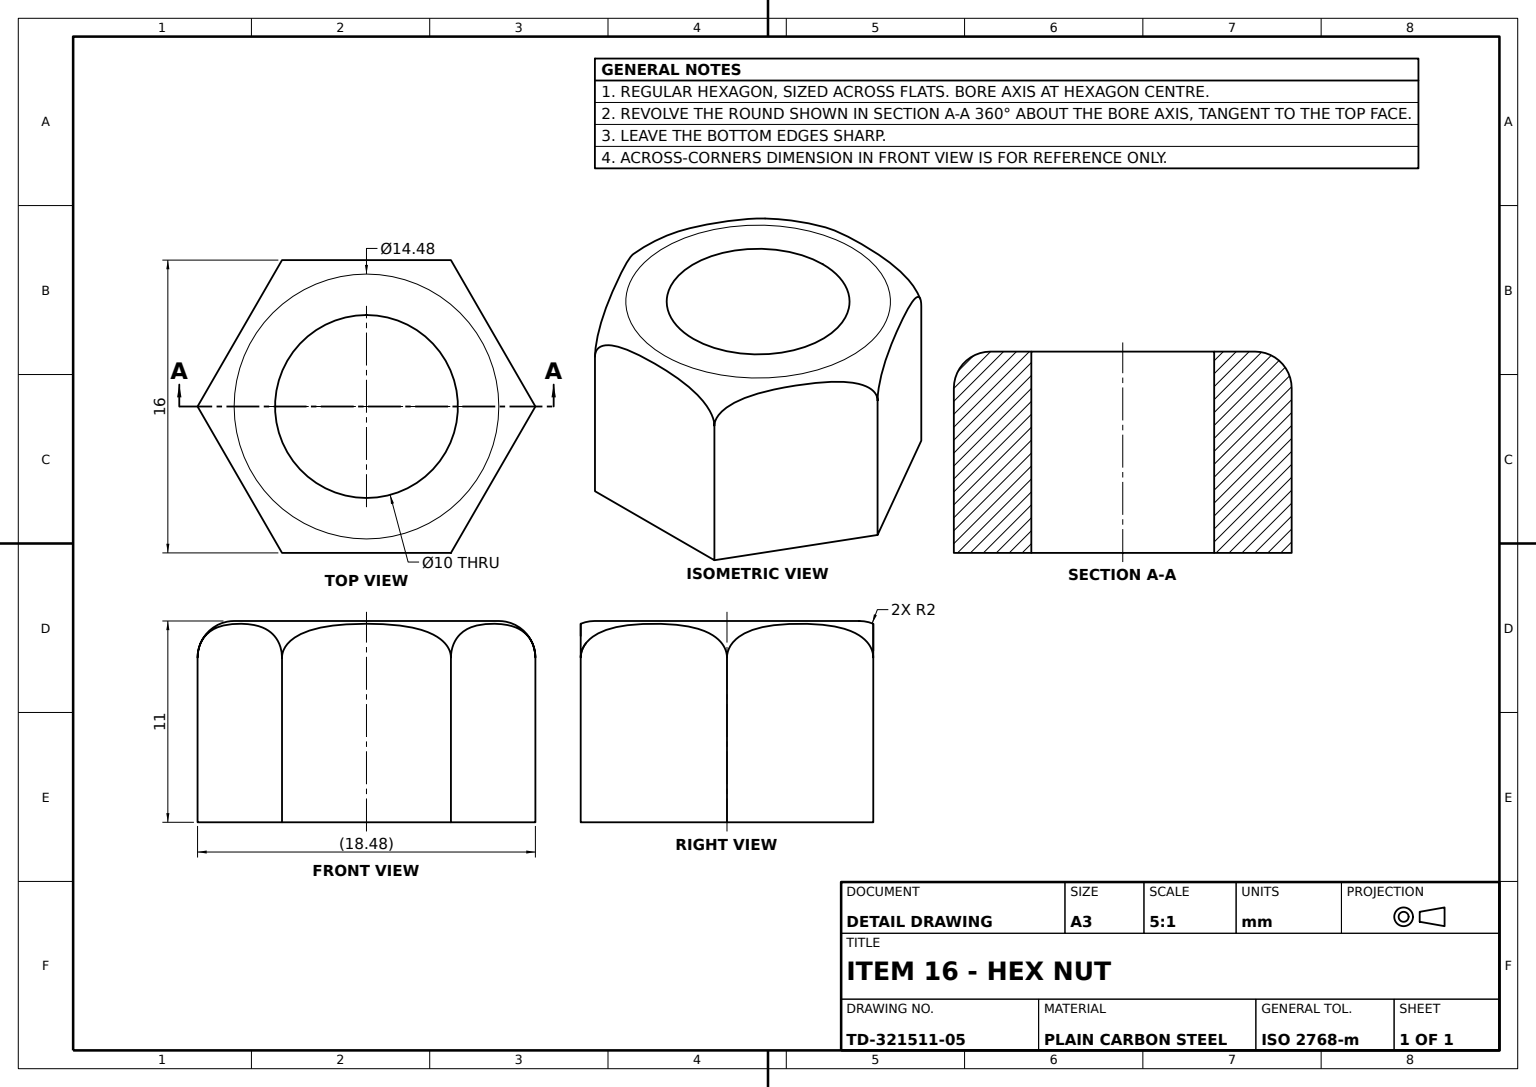
ISO-10303-21;
HEADER;
FILE_DESCRIPTION((''),'2;1');
FILE_NAME('','',(''),(''),'','','');
FILE_SCHEMA(('AUTOMOTIVE_DESIGN'));
ENDSEC;
DATA;
#1=APPLICATION_CONTEXT('');
#2=PRODUCT_CONTEXT('',#1,'mechanical');
#3=PRODUCT('','','',(#2));
#4=PRODUCT_DEFINITION_FORMATION('','',#3);
#5=PRODUCT_DEFINITION_CONTEXT('',#1,'design');
#6=PRODUCT_DEFINITION('','',#4,#5);
#7=PRODUCT_DEFINITION_SHAPE('','',#6);
#8=(LENGTH_UNIT()NAMED_UNIT(*)SI_UNIT(.MILLI.,.METRE.));
#9=(NAMED_UNIT(*)PLANE_ANGLE_UNIT()SI_UNIT($,.RADIAN.));
#10=(NAMED_UNIT(*)SI_UNIT($,.STERADIAN.)SOLID_ANGLE_UNIT());
#11=UNCERTAINTY_MEASURE_WITH_UNIT(LENGTH_MEASURE(1.E-05),#8,'distance_accuracy_value','');
#12=(GEOMETRIC_REPRESENTATION_CONTEXT(3)GLOBAL_UNCERTAINTY_ASSIGNED_CONTEXT((#11))GLOBAL_UNIT_ASSIGNED_CONTEXT((#8,#9,#10))REPRESENTATION_CONTEXT('',''));
#13=CARTESIAN_POINT('',(4.618802,3.5,8.));
#14=VERTEX_POINT('',#13);
#15=CARTESIAN_POINT('',(4.618802,-5.5,8.));
#16=VERTEX_POINT('',#15);
#17=CARTESIAN_POINT('',(4.618802,5.5,8.));
#18=DIRECTION('',(0.,-1.,0.));
#19=VECTOR('',#18,1000.);
#20=LINE('',#17,#19);
#21=EDGE_CURVE('',#14,#16,#20,.T.);
#22=ORIENTED_EDGE('',*,*,#21,.T.);
#23=CARTESIAN_POINT('',(9.237604,-5.5,0.));
#24=VERTEX_POINT('',#23);
#25=DIRECTION('',(0.5,0.,-0.866025404));
#26=VECTOR('',#25,1000.);
#27=LINE('',#15,#26);
#28=EDGE_CURVE('',#16,#24,#27,.T.);
#29=ORIENTED_EDGE('',*,*,#28,.T.);
#30=CARTESIAN_POINT('',(9.237604,3.5,0.));
#31=VERTEX_POINT('',#30);
#32=CARTESIAN_POINT('',(9.237604,5.5,0.));
#33=LINE('',#32,#19);
#34=EDGE_CURVE('',#31,#24,#33,.T.);
#35=ORIENTED_EDGE('',*,*,#34,.F.);
#36=CARTESIAN_POINT('',(9.237604,3.729784,0.));
#37=CARTESIAN_POINT('',(9.196779,3.950031,0.070712));
#38=CARTESIAN_POINT('',(9.066014,4.325166,0.297203));
#39=CARTESIAN_POINT('',(8.97987,4.47676,0.446409));
#40=CARTESIAN_POINT('',(8.790915,4.728162,0.773688));
#41=CARTESIAN_POINT('',(8.689586,4.826135,0.949196));
#42=CARTESIAN_POINT('',(8.478741,4.988958,1.31439));
#43=CARTESIAN_POINT('',(8.369616,5.052771,1.5034));
#44=CARTESIAN_POINT('',(8.042347,5.206795,2.070246));
#45=CARTESIAN_POINT('',(7.82086,5.263287,2.453872));
#46=CARTESIAN_POINT('',(7.374918,5.334811,3.226267));
#47=CARTESIAN_POINT('',(7.149945,5.349106,3.615931));
#48=CARTESIAN_POINT('',(6.701263,5.348866,4.393073));
#49=CARTESIAN_POINT('',(6.477227,5.33446,4.781114));
#50=CARTESIAN_POINT('',(6.030087,5.262072,5.555583));
#51=CARTESIAN_POINT('',(5.806107,5.20426,5.943527));
#52=CARTESIAN_POINT('',(5.478846,5.048394,6.510361));
#53=CARTESIAN_POINT('',(5.370421,4.984179,6.698159));
#54=CARTESIAN_POINT('',(5.161166,4.820901,7.060599));
#55=CARTESIAN_POINT('',(5.060602,4.722754,7.23478));
#56=CARTESIAN_POINT('',(4.919985,4.533983,7.478335));
#57=CARTESIAN_POINT('',(4.875247,4.464361,7.555825));
#58=CARTESIAN_POINT('',(4.793239,4.310754,7.697867));
#59=CARTESIAN_POINT('',(4.755308,4.225352,7.763566));
#60=CARTESIAN_POINT('',(4.659228,3.947139,7.92998));
#61=CARTESIAN_POINT('',(4.618802,3.728138,8.));
#62=B_SPLINE_CURVE_WITH_KNOTS('',3,(#30,#36,#37,#38,#39,#40,#41,#42,#43,#44,#45,#46,#47,#48,#49,#50,#51,#52,#53,#54,#55,#56,#57,#58,#59,#60,#61,#13),.UNSPECIFIED.,.F.,.F.,(4,2,2,2,2,2,2,2,2,2,2,2,2,4),(0.000000197,0.00067912,0.001358043,0.002036966,0.00271589,0.004073736,0.005431582,0.006789429,0.008147275,0.008826198,0.009505121,0.009844583,0.010184044,0.010862968),.UNSPECIFIED.);
#63=EDGE_CURVE('',#31,#14,#62,.T.);
#64=ORIENTED_EDGE('',*,*,#63,.T.);
#65=EDGE_LOOP('',(#22,#29,#35,#64));
#66=FACE_OUTER_BOUND('',#65,.T.);
#67=DIRECTION('',(-0.866025404,0.,-0.5));
#68=DIRECTION('',(-0.5,0.,0.866025404));
#69=AXIS2_PLACEMENT_3D('',#17,#67,#68);
#70=PLANE('',#69);
#71=ADVANCED_FACE('',(#66),#70,.F.);
#72=CARTESIAN_POINT('',(0.,5.348987,8.));
#73=VERTEX_POINT('',#72);
#74=CARTESIAN_POINT('',(4.618802,3.61247,8.));
#75=CARTESIAN_POINT('',(4.599021,3.726679,8.));
#76=CARTESIAN_POINT('',(4.525978,3.940566,8.));
#77=CARTESIAN_POINT('',(4.47223,4.042759,8.));
#78=CARTESIAN_POINT('',(4.27939,4.320531,8.));
#79=CARTESIAN_POINT('',(4.106464,4.473927,8.));
#80=CARTESIAN_POINT('',(3.733342,4.723624,8.));
#81=CARTESIAN_POINT('',(3.527968,4.823675,8.));
#82=CARTESIAN_POINT('',(3.109536,4.986128,8.));
#83=CARTESIAN_POINT('',(2.89499,5.049417,8.));
#84=CARTESIAN_POINT('',(2.241083,5.204726,8.));
#85=CARTESIAN_POINT('',(1.792291,5.262523,8.));
#86=CARTESIAN_POINT('',(0.898193,5.33463,8.));
#87=CARTESIAN_POINT('',(0.44959,5.348987,8.));
#88=B_SPLINE_CURVE_WITH_KNOTS('',3,(#13,#74,#75,#76,#77,#78,#79,#80,#81,#82,#83,#84,#85,#86,#87,#72),.UNSPECIFIED.,.F.,.F.,(4,2,2,2,2,2,2,4),(0.01622008,0.01655642,0.016892761,0.017565443,0.018238124,0.018910806,0.020256169,0.021601532),.UNSPECIFIED.);
#89=EDGE_CURVE('',#14,#73,#88,.T.);
#90=ORIENTED_EDGE('',*,*,#89,.T.);
#91=CARTESIAN_POINT('',(-4.618802,3.5,8.));
#92=VERTEX_POINT('',#91);
#93=CARTESIAN_POINT('',(-0.449879,5.348987,8.));
#94=CARTESIAN_POINT('',(-0.898734,5.334614,8.));
#95=CARTESIAN_POINT('',(-1.79335,5.26241,8.));
#96=CARTESIAN_POINT('',(-2.241963,5.204672,8.));
#97=CARTESIAN_POINT('',(-2.89755,5.048731,8.));
#98=CARTESIAN_POINT('',(-3.112992,4.985099,8.));
#99=CARTESIAN_POINT('',(-3.534111,4.820971,8.));
#100=CARTESIAN_POINT('',(-3.73565,4.722413,8.));
#101=CARTESIAN_POINT('',(-4.10914,4.471797,8.));
#102=CARTESIAN_POINT('',(-4.280837,4.319457,8.));
#103=CARTESIAN_POINT('',(-4.47453,4.038929,8.));
#104=CARTESIAN_POINT('',(-4.526633,3.939248,8.));
#105=CARTESIAN_POINT('',(-4.599587,3.724409,8.));
#106=CARTESIAN_POINT('',(-4.618802,3.61247,8.));
#107=B_SPLINE_CURVE_WITH_KNOTS('',3,(#72,#93,#94,#95,#96,#97,#98,#99,#100,#101,#102,#103,#104,#105,#106,#91),.UNSPECIFIED.,.F.,.F.,(4,2,2,2,2,2,2,4),(0.,0.001346227,0.002692455,0.003365569,0.004038682,0.004711796,0.005048353,0.00538491),.UNSPECIFIED.);
#108=EDGE_CURVE('',#73,#92,#107,.T.);
#109=ORIENTED_EDGE('',*,*,#108,.T.);
#110=CARTESIAN_POINT('',(-4.618802,-5.5,8.));
#111=VERTEX_POINT('',#110);
#112=CARTESIAN_POINT('',(-4.618802,5.5,8.));
#113=LINE('',#112,#19);
#114=EDGE_CURVE('',#92,#111,#113,.T.);
#115=ORIENTED_EDGE('',*,*,#114,.T.);
#116=DIRECTION('',(1.,0.,0.));
#117=VECTOR('',#116,1000.);
#118=LINE('',#110,#117);
#119=EDGE_CURVE('',#111,#16,#118,.T.);
#120=ORIENTED_EDGE('',*,*,#119,.T.);
#121=ORIENTED_EDGE('',*,*,#21,.F.);
#122=EDGE_LOOP('',(#90,#109,#115,#120,#121));
#123=FACE_OUTER_BOUND('',#122,.T.);
#124=DIRECTION('',(0.,0.,-1.));
#125=DIRECTION('',(-1.,0.,0.));
#126=AXIS2_PLACEMENT_3D('',#112,#124,#125);
#127=PLANE('',#126);
#128=ADVANCED_FACE('',(#123),#127,.F.);
#129=ORIENTED_EDGE('',*,*,#34,.T.);
#130=CARTESIAN_POINT('',(4.618802,-5.5,-8.));
#131=VERTEX_POINT('',#130);
#132=DIRECTION('',(-0.5,0.,-0.866025404));
#133=VECTOR('',#132,1000.);
#134=LINE('',#23,#133);
#135=EDGE_CURVE('',#24,#131,#134,.T.);
#136=ORIENTED_EDGE('',*,*,#135,.T.);
#137=CARTESIAN_POINT('',(4.618802,3.5,-8.));
#138=VERTEX_POINT('',#137);
#139=CARTESIAN_POINT('',(4.618802,5.5,-8.));
#140=LINE('',#139,#19);
#141=EDGE_CURVE('',#138,#131,#140,.T.);
#142=ORIENTED_EDGE('',*,*,#141,.F.);
#143=CARTESIAN_POINT('',(4.618802,3.729784,-8.));
#144=CARTESIAN_POINT('',(4.659628,3.950031,-7.929288));
#145=CARTESIAN_POINT('',(4.790393,4.325166,-7.702797));
#146=CARTESIAN_POINT('',(4.876537,4.47676,-7.553591));
#147=CARTESIAN_POINT('',(5.065491,4.728162,-7.226312));
#148=CARTESIAN_POINT('',(5.166821,4.826135,-7.050804));
#149=CARTESIAN_POINT('',(5.377665,4.988958,-6.68561));
#150=CARTESIAN_POINT('',(5.48679,5.052771,-6.4966));
#151=CARTESIAN_POINT('',(5.814059,5.206795,-5.929754));
#152=CARTESIAN_POINT('',(6.035546,5.263287,-5.546128));
#153=CARTESIAN_POINT('',(6.481488,5.334811,-4.773733));
#154=CARTESIAN_POINT('',(6.706461,5.349106,-4.384069));
#155=CARTESIAN_POINT('',(7.155144,5.348866,-3.606927));
#156=CARTESIAN_POINT('',(7.37918,5.33446,-3.218886));
#157=CARTESIAN_POINT('',(7.826319,5.262072,-2.444417));
#158=CARTESIAN_POINT('',(8.050299,5.20426,-2.056473));
#159=CARTESIAN_POINT('',(8.377561,5.048394,-1.489639));
#160=CARTESIAN_POINT('',(8.485986,4.984179,-1.301841));
#161=CARTESIAN_POINT('',(8.695241,4.820901,-0.939401));
#162=CARTESIAN_POINT('',(8.795804,4.722754,-0.76522));
#163=CARTESIAN_POINT('',(8.936421,4.533983,-0.521665));
#164=CARTESIAN_POINT('',(8.98116,4.464361,-0.444175));
#165=CARTESIAN_POINT('',(9.063168,4.310754,-0.302133));
#166=CARTESIAN_POINT('',(9.101099,4.225352,-0.236434));
#167=CARTESIAN_POINT('',(9.197178,3.947139,-0.07002));
#168=CARTESIAN_POINT('',(9.237604,3.728138,0.));
#169=B_SPLINE_CURVE_WITH_KNOTS('',3,(#137,#143,#144,#145,#146,#147,#148,#149,#150,#151,#152,#153,#154,#155,#156,#157,#158,#159,#160,#161,#162,#163,#164,#165,#166,#167,#168,#30),.UNSPECIFIED.,.F.,.F.,(4,2,2,2,2,2,2,2,2,2,2,2,2,4),(0.000000197,0.00067912,0.001358043,0.002036966,0.00271589,0.004073736,0.005431582,0.006789429,0.008147275,0.008826198,0.009505121,0.009844583,0.010184044,0.010862968),.UNSPECIFIED.);
#170=EDGE_CURVE('',#138,#31,#169,.T.);
#171=ORIENTED_EDGE('',*,*,#170,.T.);
#172=EDGE_LOOP('',(#129,#136,#142,#171));
#173=FACE_OUTER_BOUND('',#172,.T.);
#174=DIRECTION('',(-0.866025404,0.,0.5));
#175=DIRECTION('',(0.5,0.,0.866025404));
#176=AXIS2_PLACEMENT_3D('',#32,#174,#175);
#177=PLANE('',#176);
#178=ADVANCED_FACE('',(#173),#177,.F.);
#179=CARTESIAN_POINT('',(0.,5.348987,-8.));
#180=VERTEX_POINT('',#179);
#181=CARTESIAN_POINT('',(0.449879,5.348987,-8.));
#182=CARTESIAN_POINT('',(0.898734,5.334614,-8.));
#183=CARTESIAN_POINT('',(1.79335,5.26241,-8.));
#184=CARTESIAN_POINT('',(2.241963,5.204672,-8.));
#185=CARTESIAN_POINT('',(2.89755,5.048731,-8.));
#186=CARTESIAN_POINT('',(3.112992,4.985099,-8.));
#187=CARTESIAN_POINT('',(3.534111,4.820971,-8.));
#188=CARTESIAN_POINT('',(3.73565,4.722413,-8.));
#189=CARTESIAN_POINT('',(4.10914,4.471797,-8.));
#190=CARTESIAN_POINT('',(4.280837,4.319457,-8.));
#191=CARTESIAN_POINT('',(4.47453,4.038929,-8.));
#192=CARTESIAN_POINT('',(4.526633,3.939248,-8.));
#193=CARTESIAN_POINT('',(4.599587,3.724409,-8.));
#194=CARTESIAN_POINT('',(4.618802,3.61247,-8.));
#195=B_SPLINE_CURVE_WITH_KNOTS('',3,(#179,#181,#182,#183,#184,#185,#186,#187,#188,#189,#190,#191,#192,#193,#194,#137),.UNSPECIFIED.,.F.,.F.,(4,2,2,2,2,2,2,4),(0.,0.001346227,0.002692455,0.003365569,0.004038682,0.004711796,0.005048353,0.00538491),.UNSPECIFIED.);
#196=EDGE_CURVE('',#180,#138,#195,.T.);
#197=ORIENTED_EDGE('',*,*,#196,.T.);
#198=ORIENTED_EDGE('',*,*,#141,.T.);
#199=CARTESIAN_POINT('',(-4.618802,-5.5,-8.));
#200=VERTEX_POINT('',#199);
#201=VECTOR('',#125,1000.);
#202=LINE('',#130,#201);
#203=EDGE_CURVE('',#131,#200,#202,.T.);
#204=ORIENTED_EDGE('',*,*,#203,.T.);
#205=CARTESIAN_POINT('',(-4.618802,3.5,-8.));
#206=VERTEX_POINT('',#205);
#207=CARTESIAN_POINT('',(-4.618802,5.5,-8.));
#208=LINE('',#207,#19);
#209=EDGE_CURVE('',#206,#200,#208,.T.);
#210=ORIENTED_EDGE('',*,*,#209,.F.);
#211=CARTESIAN_POINT('',(-4.618802,3.61247,-8.));
#212=CARTESIAN_POINT('',(-4.599021,3.726679,-8.));
#213=CARTESIAN_POINT('',(-4.525978,3.940566,-8.));
#214=CARTESIAN_POINT('',(-4.47223,4.042759,-8.));
#215=CARTESIAN_POINT('',(-4.27939,4.320531,-8.));
#216=CARTESIAN_POINT('',(-4.106464,4.473927,-8.));
#217=CARTESIAN_POINT('',(-3.733342,4.723624,-8.));
#218=CARTESIAN_POINT('',(-3.527968,4.823675,-8.));
#219=CARTESIAN_POINT('',(-3.109536,4.986128,-8.));
#220=CARTESIAN_POINT('',(-2.89499,5.049417,-8.));
#221=CARTESIAN_POINT('',(-2.241083,5.204726,-8.));
#222=CARTESIAN_POINT('',(-1.792291,5.262523,-8.));
#223=CARTESIAN_POINT('',(-0.898193,5.33463,-8.));
#224=CARTESIAN_POINT('',(-0.44959,5.348987,-8.));
#225=B_SPLINE_CURVE_WITH_KNOTS('',3,(#205,#211,#212,#213,#214,#215,#216,#217,#218,#219,#220,#221,#222,#223,#224,#179),.UNSPECIFIED.,.F.,.F.,(4,2,2,2,2,2,2,4),(0.01622008,0.01655642,0.016892761,0.017565443,0.018238124,0.018910806,0.020256169,0.021601532),.UNSPECIFIED.);
#226=EDGE_CURVE('',#206,#180,#225,.T.);
#227=ORIENTED_EDGE('',*,*,#226,.T.);
#228=EDGE_LOOP('',(#197,#198,#204,#210,#227));
#229=FACE_OUTER_BOUND('',#228,.T.);
#230=DIRECTION('',(0.,0.,1.));
#231=AXIS2_PLACEMENT_3D('',#139,#230,#116);
#232=PLANE('',#231);
#233=ADVANCED_FACE('',(#229),#232,.F.);
#234=CARTESIAN_POINT('',(0.,5.5,7.237604));
#235=VERTEX_POINT('',#234);
#236=CARTESIAN_POINT('',(0.,5.5,-7.237604));
#237=VERTEX_POINT('',#236);
#238=CARTESIAN_POINT('',(0.,5.5,0.));
#239=AXIS2_PLACEMENT_3D('',#238,#18,#124);
#240=CIRCLE('',#239,7.237604);
#241=EDGE_CURVE('',#235,#237,#240,.T.);
#242=ORIENTED_EDGE('',*,*,#241,.T.);
#243=CARTESIAN_POINT('',(0.,3.5,-7.237604));
#244=AXIS2_PLACEMENT_3D('',#243,#125,#230);
#245=CIRCLE('',#244,2.);
#246=EDGE_CURVE('',#237,#180,#245,.T.);
#247=ORIENTED_EDGE('',*,*,#246,.T.);
#248=ORIENTED_EDGE('',*,*,#226,.F.);
#249=CARTESIAN_POINT('',(-9.237604,3.5,0.));
#250=VERTEX_POINT('',#249);
#251=CARTESIAN_POINT('',(-9.237604,3.729784,0.));
#252=CARTESIAN_POINT('',(-9.196779,3.950031,-0.070712));
#253=CARTESIAN_POINT('',(-9.066014,4.325166,-0.297203));
#254=CARTESIAN_POINT('',(-8.97987,4.47676,-0.446409));
#255=CARTESIAN_POINT('',(-8.790915,4.728162,-0.773688));
#256=CARTESIAN_POINT('',(-8.689586,4.826135,-0.949196));
#257=CARTESIAN_POINT('',(-8.478741,4.988958,-1.31439));
#258=CARTESIAN_POINT('',(-8.369616,5.052771,-1.5034));
#259=CARTESIAN_POINT('',(-8.042347,5.206795,-2.070246));
#260=CARTESIAN_POINT('',(-7.82086,5.263287,-2.453872));
#261=CARTESIAN_POINT('',(-7.374918,5.334811,-3.226267));
#262=CARTESIAN_POINT('',(-7.149945,5.349106,-3.615931));
#263=CARTESIAN_POINT('',(-6.701263,5.348866,-4.393073));
#264=CARTESIAN_POINT('',(-6.477227,5.33446,-4.781114));
#265=CARTESIAN_POINT('',(-6.030087,5.262072,-5.555583));
#266=CARTESIAN_POINT('',(-5.806107,5.20426,-5.943527));
#267=CARTESIAN_POINT('',(-5.478846,5.048394,-6.510361));
#268=CARTESIAN_POINT('',(-5.370421,4.984179,-6.698159));
#269=CARTESIAN_POINT('',(-5.161166,4.820901,-7.060599));
#270=CARTESIAN_POINT('',(-5.060602,4.722754,-7.23478));
#271=CARTESIAN_POINT('',(-4.919985,4.533983,-7.478335));
#272=CARTESIAN_POINT('',(-4.875247,4.464361,-7.555825));
#273=CARTESIAN_POINT('',(-4.793239,4.310754,-7.697867));
#274=CARTESIAN_POINT('',(-4.755308,4.225352,-7.763566));
#275=CARTESIAN_POINT('',(-4.659228,3.947139,-7.92998));
#276=CARTESIAN_POINT('',(-4.618802,3.728138,-8.));
#277=B_SPLINE_CURVE_WITH_KNOTS('',3,(#249,#251,#252,#253,#254,#255,#256,#257,#258,#259,#260,#261,#262,#263,#264,#265,#266,#267,#268,#269,#270,#271,#272,#273,#274,#275,#276,#205),.UNSPECIFIED.,.F.,.F.,(4,2,2,2,2,2,2,2,2,2,2,2,2,4),(0.000000197,0.00067912,0.001358043,0.002036966,0.00271589,0.004073736,0.005431582,0.006789429,0.008147275,0.008826198,0.009505121,0.009844583,0.010184044,0.010862968),.UNSPECIFIED.);
#278=EDGE_CURVE('',#250,#206,#277,.T.);
#279=ORIENTED_EDGE('',*,*,#278,.F.);
#280=CARTESIAN_POINT('',(-4.618802,3.729784,8.));
#281=CARTESIAN_POINT('',(-4.659628,3.950031,7.929288));
#282=CARTESIAN_POINT('',(-4.790393,4.325166,7.702797));
#283=CARTESIAN_POINT('',(-4.876537,4.47676,7.553591));
#284=CARTESIAN_POINT('',(-5.065491,4.728162,7.226312));
#285=CARTESIAN_POINT('',(-5.166821,4.826135,7.050804));
#286=CARTESIAN_POINT('',(-5.377665,4.988958,6.68561));
#287=CARTESIAN_POINT('',(-5.48679,5.052771,6.4966));
#288=CARTESIAN_POINT('',(-5.814059,5.206795,5.929754));
#289=CARTESIAN_POINT('',(-6.035546,5.263287,5.546128));
#290=CARTESIAN_POINT('',(-6.481488,5.334811,4.773733));
#291=CARTESIAN_POINT('',(-6.706461,5.349106,4.384069));
#292=CARTESIAN_POINT('',(-7.155144,5.348866,3.606927));
#293=CARTESIAN_POINT('',(-7.37918,5.33446,3.218886));
#294=CARTESIAN_POINT('',(-7.826319,5.262072,2.444417));
#295=CARTESIAN_POINT('',(-8.050299,5.20426,2.056473));
#296=CARTESIAN_POINT('',(-8.377561,5.048394,1.489639));
#297=CARTESIAN_POINT('',(-8.485986,4.984179,1.301841));
#298=CARTESIAN_POINT('',(-8.695241,4.820901,0.939401));
#299=CARTESIAN_POINT('',(-8.795804,4.722754,0.76522));
#300=CARTESIAN_POINT('',(-8.936421,4.533983,0.521665));
#301=CARTESIAN_POINT('',(-8.98116,4.464361,0.444175));
#302=CARTESIAN_POINT('',(-9.063168,4.310754,0.302133));
#303=CARTESIAN_POINT('',(-9.101099,4.225352,0.236434));
#304=CARTESIAN_POINT('',(-9.197178,3.947139,0.07002));
#305=CARTESIAN_POINT('',(-9.237604,3.728138,0.));
#306=B_SPLINE_CURVE_WITH_KNOTS('',3,(#91,#280,#281,#282,#283,#284,#285,#286,#287,#288,#289,#290,#291,#292,#293,#294,#295,#296,#297,#298,#299,#300,#301,#302,#303,#304,#305,#249),.UNSPECIFIED.,.F.,.F.,(4,2,2,2,2,2,2,2,2,2,2,2,2,4),(0.000000197,0.00067912,0.001358043,0.002036966,0.00271589,0.004073736,0.005431582,0.006789429,0.008147275,0.008826198,0.009505121,0.009844583,0.010184044,0.010862968),.UNSPECIFIED.);
#307=EDGE_CURVE('',#92,#250,#306,.T.);
#308=ORIENTED_EDGE('',*,*,#307,.F.);
#309=ORIENTED_EDGE('',*,*,#108,.F.);
#310=CARTESIAN_POINT('',(0.,3.5,7.237604));
#311=AXIS2_PLACEMENT_3D('',#310,#116,#124);
#312=CIRCLE('',#311,2.);
#313=EDGE_CURVE('',#235,#73,#312,.T.);
#314=ORIENTED_EDGE('',*,*,#313,.F.);
#315=EDGE_LOOP('',(#242,#247,#248,#279,#308,#309,#314));
#316=FACE_OUTER_BOUND('',#315,.T.);
#317=CARTESIAN_POINT('',(0.,3.5,0.));
#318=AXIS2_PLACEMENT_3D('',#317,#18,#124);
#319=TOROIDAL_SURFACE('',#318,7.237604,2.);
#320=ADVANCED_FACE('',(#316),#319,.T.);
#321=ORIENTED_EDGE('',*,*,#196,.F.);
#322=ORIENTED_EDGE('',*,*,#246,.F.);
#323=EDGE_CURVE('',#237,#235,#240,.T.);
#324=ORIENTED_EDGE('',*,*,#323,.T.);
#325=ORIENTED_EDGE('',*,*,#313,.T.);
#326=ORIENTED_EDGE('',*,*,#89,.F.);
#327=ORIENTED_EDGE('',*,*,#63,.F.);
#328=ORIENTED_EDGE('',*,*,#170,.F.);
#329=EDGE_LOOP('',(#321,#322,#324,#325,#326,#327,#328));
#330=FACE_OUTER_BOUND('',#329,.T.);
#331=ADVANCED_FACE('',(#330),#319,.T.);
#332=CARTESIAN_POINT('',(-9.237604,-5.5,0.));
#333=VERTEX_POINT('',#332);
#334=VECTOR('',#68,1000.);
#335=LINE('',#199,#334);
#336=EDGE_CURVE('',#200,#333,#335,.T.);
#337=ORIENTED_EDGE('',*,*,#336,.F.);
#338=ORIENTED_EDGE('',*,*,#203,.F.);
#339=ORIENTED_EDGE('',*,*,#135,.F.);
#340=ORIENTED_EDGE('',*,*,#28,.F.);
#341=ORIENTED_EDGE('',*,*,#119,.F.);
#342=VECTOR('',#175,1000.);
#343=LINE('',#332,#342);
#344=EDGE_CURVE('',#333,#111,#343,.T.);
#345=ORIENTED_EDGE('',*,*,#344,.F.);
#346=EDGE_LOOP('',(#337,#338,#339,#340,#341,#345));
#347=FACE_OUTER_BOUND('',#346,.T.);
#348=CARTESIAN_POINT('',(0.,-5.5,5.));
#349=VERTEX_POINT('',#348);
#350=CARTESIAN_POINT('',(0.,-5.5,-5.));
#351=VERTEX_POINT('',#350);
#352=CARTESIAN_POINT('',(0.,-5.5,0.));
#353=DIRECTION('',(0.,1.,0.));
#354=AXIS2_PLACEMENT_3D('',#352,#353,#230);
#355=CIRCLE('',#354,5.);
#356=EDGE_CURVE('',#349,#351,#355,.T.);
#357=ORIENTED_EDGE('',*,*,#356,.T.);
#358=EDGE_CURVE('',#351,#349,#355,.T.);
#359=ORIENTED_EDGE('',*,*,#358,.T.);
#360=EDGE_LOOP('',(#357,#359));
#361=FACE_BOUND('',#360,.T.);
#362=PLANE('',#354);
#363=ADVANCED_FACE('',(#347,#361),#362,.F.);
#364=ORIENTED_EDGE('',*,*,#241,.F.);
#365=ORIENTED_EDGE('',*,*,#323,.F.);
#366=EDGE_LOOP('',(#364,#365));
#367=FACE_OUTER_BOUND('',#366,.T.);
#368=CARTESIAN_POINT('',(0.,5.5,-5.));
#369=VERTEX_POINT('',#368);
#370=CARTESIAN_POINT('',(0.,5.5,5.));
#371=VERTEX_POINT('',#370);
#372=AXIS2_PLACEMENT_3D('',#238,#353,#230);
#373=CIRCLE('',#372,5.);
#374=EDGE_CURVE('',#369,#371,#373,.T.);
#375=ORIENTED_EDGE('',*,*,#374,.F.);
#376=EDGE_CURVE('',#371,#369,#373,.T.);
#377=ORIENTED_EDGE('',*,*,#376,.F.);
#378=EDGE_LOOP('',(#375,#377));
#379=FACE_BOUND('',#378,.T.);
#380=PLANE('',#372);
#381=ADVANCED_FACE('',(#367,#379),#380,.T.);
#382=ORIENTED_EDGE('',*,*,#114,.F.);
#383=ORIENTED_EDGE('',*,*,#307,.T.);
#384=CARTESIAN_POINT('',(-9.237604,5.5,0.));
#385=LINE('',#384,#19);
#386=EDGE_CURVE('',#250,#333,#385,.T.);
#387=ORIENTED_EDGE('',*,*,#386,.T.);
#388=ORIENTED_EDGE('',*,*,#344,.T.);
#389=EDGE_LOOP('',(#382,#383,#387,#388));
#390=FACE_OUTER_BOUND('',#389,.T.);
#391=DIRECTION('',(0.866025404,0.,-0.5));
#392=AXIS2_PLACEMENT_3D('',#384,#391,#132);
#393=PLANE('',#392);
#394=ADVANCED_FACE('',(#390),#393,.F.);
#395=ORIENTED_EDGE('',*,*,#386,.F.);
#396=ORIENTED_EDGE('',*,*,#278,.T.);
#397=ORIENTED_EDGE('',*,*,#209,.T.);
#398=ORIENTED_EDGE('',*,*,#336,.T.);
#399=EDGE_LOOP('',(#395,#396,#397,#398));
#400=FACE_OUTER_BOUND('',#399,.T.);
#401=DIRECTION('',(0.866025404,0.,0.5));
#402=AXIS2_PLACEMENT_3D('',#207,#401,#25);
#403=PLANE('',#402);
#404=ADVANCED_FACE('',(#400),#403,.F.);
#405=ORIENTED_EDGE('',*,*,#376,.T.);
#406=VECTOR('',#353,1000.);
#407=LINE('',#350,#406);
#408=EDGE_CURVE('',#351,#369,#407,.T.);
#409=ORIENTED_EDGE('',*,*,#408,.F.);
#410=ORIENTED_EDGE('',*,*,#356,.F.);
#411=LINE('',#348,#406);
#412=EDGE_CURVE('',#349,#371,#411,.T.);
#413=ORIENTED_EDGE('',*,*,#412,.T.);
#414=EDGE_LOOP('',(#405,#409,#410,#413));
#415=FACE_OUTER_BOUND('',#414,.T.);
#416=CYLINDRICAL_SURFACE('',#354,5.);
#417=ADVANCED_FACE('',(#415),#416,.F.);
#418=ORIENTED_EDGE('',*,*,#358,.F.);
#419=ORIENTED_EDGE('',*,*,#408,.T.);
#420=ORIENTED_EDGE('',*,*,#374,.T.);
#421=ORIENTED_EDGE('',*,*,#412,.F.);
#422=EDGE_LOOP('',(#418,#419,#420,#421));
#423=FACE_OUTER_BOUND('',#422,.T.);
#424=ADVANCED_FACE('',(#423),#416,.F.);
#425=CLOSED_SHELL('',(#71,#128,#178,#233,#320,#331,#363,#381,#394,#404,#417,#424));
#426=MANIFOLD_SOLID_BREP('',#425);
#427=ADVANCED_BREP_SHAPE_REPRESENTATION('',(#426),#12);
#428=SHAPE_DEFINITION_REPRESENTATION(#7,#427);
ENDSEC;
END-ISO-10303-21;
